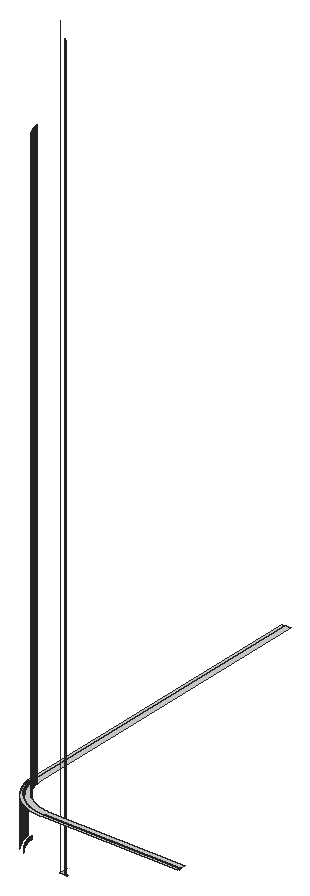
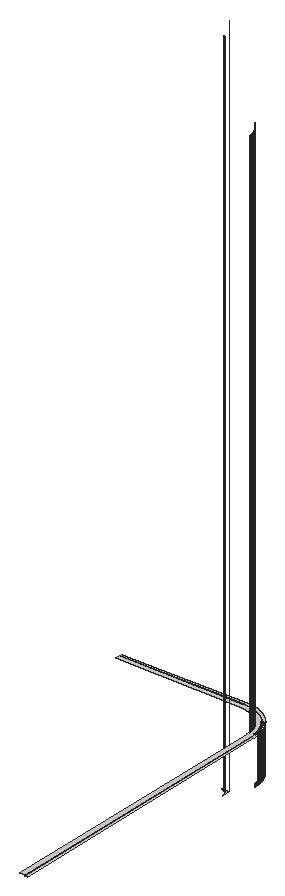
# SketchUp Ruby script. Lengths in inches.
U = 1.inch
M = Sketchup.active_model
def pt(a) = Geom::Point3d.new(a.map { |v| v * U })
def face(e, loops, mat)
  f = e.add_face(loops[0].map { |a| pt(a) })
  loops[1..].each { |l| e.add_face(l.map { |a| pt(a) }).erase! }
  f.material = f.back_material = mat if mat
  f
end
# faces: each face lists its corners as indices into pts; further lists are holes
def faces(e, pts, list, mat = nil) = list.each { |f| face(e, (f[0].is_a?(Array) ? f : [f]).map { |l| l.map { |i| pts[i] } }, mat) }
# xy, xz, yz: faces in a plane at the given z, y or x. An outline is a flat list of corners, or four numbers for a rectangle; further outlines are holes
def ring(l) = l.size == 4 ? [[l[0], l[1]], [l[2], l[1]], [l[2], l[3]], [l[0], l[3]]] : l.each_slice(2).to_a
def flat(e, list, mat, &to3) = list.each { |f| face(e, (f[0].is_a?(Array) ? f : [f]).map { |l| ring(l).map { |u, v| to3.(u, v) } }, mat) }
def xy(e, z, list, mat = nil) = flat(e, list, mat) { |x, y| [x, y, z] }
def xz(e, y, list, mat = nil) = flat(e, list, mat) { |x, z| [x, y, z] }
def yz(e, x, list, mat = nil) = flat(e, list, mat) { |y, z| [x, y, z] }
def lines(e, pts, list) = list.each { |a, b| e.add_line(pt(pts[a]), pt(pts[b])) }
# prism: a flat outline (further loops are holes) pulled along v
def prism(e, loops, v, mat = nil)
  f = face(e, loops, mat); d = Geom::Vector3d.new(v.map { |x| x * U })
  f.pushpull(f.normal.samedirection?(d) ? d.length : -d.length)
end
def box(e, o, s, mat = nil) = prism(e, [[o, [o[0] + s[0], o[1], o[2]], [o[0] + s[0], o[1] + s[1], o[2]], [o[0], o[1] + s[1], o[2]]]], [0, 0, s[2]], mat)
def at(x, y, z, deg = 0) = Geom::Transformation.translation(pt([x, y, z])) * Geom::Transformation.rotation(ORIGIN, Z_AXIS, deg.degrees)
def axes(o, x, y, z) = Geom::Transformation.new([*x, 0, *y, 0, *z, 0, *pt(o).to_a, 1])
def part(name) = M.definitions.add(name)
# library, detail: a bought-in or finely detailed component or shape, given as its bounding box
def library(name, o, s) = part(name).tap { |d| box(d.entities, o, s) }
def detail(e, o, s) = box(e.add_group.entities, o, s)
def put(e, d, t, mat = nil) = e.add_instance(d, t).tap { |i| i.material = mat if mat }
def group(e, t, mat = nil) = e.add_group.tap { |g| g.transformation = t; g.material = mat if mat }.entities
root = M.entities
M.materials.add("[Quartz Light Brown]").color = [215, 212, 212]
xy(root,126,[[213,155,213.001,157.921,213.002,157.882,213.002,157.881,213.004,157.843,213.006,157.804,213.009,157.765,213.013,157.725,213.016,157.686,213.026,157.608,213.031,157.57,213.043,157.492,213.05,157.453,213.058,157.415,213.066,157.376,213.074,157.338,213.092,157.262,213.102,157.224,213.135,157.11,213.159,157.036,213.185,156.962,213.199,156.925,213.214,156.888,213.228,156.852,213.244,156.816,213.259,156.78,213.276,156.744,213.292,156.708,213.309,156.673,213.345,156.603,213.364,156.569,213.383,156.534,213.402,156.5,213.422,156.466,213.442,156.433,213.463,156.399,213.484,156.366,213.506,156.333,213.55,156.269,213.596,156.205,213.644,156.143,213.669,156.112,213.693,156.082,213.719,156.052,213.744,156.022,213.771,155.993,213.796,155.964,213.797,155.964,213.824,155.935,213.851,155.907,213.907,155.851,213.935,155.824,213.963,155.798,213.964,155.797,213.993,155.771,214.022,155.744,214.051,155.72,214.052,155.719,214.082,155.693,214.112,155.669,214.141,155.645,214.143,155.644,214.205,155.596,214.235,155.574,214.237,155.573,214.269,155.55,214.301,155.528,214.332,155.507,214.333,155.506,214.366,155.484,214.399,155.463,214.431,155.443,214.433,155.442,214.466,155.422,214.5,155.402,214.532,155.384,214.534,155.383,214.569,155.364,214.603,155.345,214.636,155.328,214.638,155.327,214.673,155.309,214.708,155.292,214.742,155.277,214.744,155.276,214.78,155.259,214.816,155.244,214.85,155.229,214.852,155.228,214.888,155.214,214.925,155.199,214.959,155.186,214.962,155.185,215.036,155.159,215.07,155.148,215.073,155.147,215.11,155.135,215.148,155.124,215.183,155.113,215.186,155.113,215.224,155.102,215.262,155.092,215.297,155.084,215.3,155.083,215.338,155.074,215.376,155.066,215.412,155.058,215.415,155.058,215.453,155.05,215.492,155.043,215.528,155.037,215.531,155.037,215.57,155.031,215.608,155.026,215.644,155.021,215.647,155.021,215.686,155.016,215.725,155.013,215.761,155.01,215.765,155.009,215.804,155.006,215.843,155.004,215.879,155.002,215.882,155.002,215.921,155.001]],"[Quartz Light Brown]")
xy(root,149.75,[[216,143.75,263.5,143.75,263.5,144.25,216,144.25,215.82,144.251,215.64,144.255,215.46,144.261,215.28,144.269,215.101,144.279,214.921,144.292,214.742,144.308,214.563,144.325,214.384,144.345,214.205,144.368,214.027,144.392,213.849,144.419,213.671,144.449,213.494,144.48,213.318,144.514,213.141,144.55,212.965,144.589,212.79,144.63,212.615,144.673,212.441,144.719,212.268,144.766,212.095,144.816,211.923,144.868,211.751,144.923,211.58,144.98,211.41,145.039,211.241,145.1,211.072,145.163,210.905,145.229,210.738,145.297,210.572,145.367,210.407,145.439,210.243,145.513,210.08,145.589,209.919,145.668,209.758,145.749,209.598,145.831,209.439,145.916,209.281,146.003,209.125,146.092,208.97,146.183,208.816,146.276,208.663,146.371,208.511,146.468,208.361,146.567,208.212,146.668,208.064,146.771,207.918,146.876,207.773,146.983,207.63,147.091,207.487,147.202,207.347,147.314,207.208,147.428,207.07,147.544,206.934,147.662,206.799,147.782,206.666,147.903,206.535,148.026,206.405,148.151,206.277,148.277,206.151,148.405,206.026,148.535,205.903,148.666,205.782,148.799,205.662,148.934,205.544,149.07,205.428,149.208,205.314,149.347,205.202,149.487,205.091,149.63,204.983,149.773,204.876,149.918,204.771,150.064,204.668,150.212,204.567,150.361,204.468,150.511,204.371,150.663,204.276,150.816,204.183,150.97,204.092,151.125,204.003,151.281,203.916,151.439,203.831,151.598,203.749,151.758,203.668,151.919,203.589,152.08,203.513,152.243,203.439,152.407,203.367,152.572,203.297,152.738,203.229,152.905,203.163,153.072,203.1,153.241,203.039,153.41,202.98,153.58,202.923,153.751,202.868,153.923,202.816,154.095,202.766,154.268,202.719,154.441,202.673,154.615,202.63,154.79,202.589,154.965,202.55,155.141,202.514,155.318,202.48,155.494,202.449,155.671,202.419,155.849,202.392,156.027,202.368,156.205,202.345,156.384,202.325,156.563,202.308,156.742,202.292,156.921,202.279,157.101,202.269,157.28,202.261,157.46,202.255,157.64,202.251,157.82,202.25,158,202.25,266,201.75,266,201.75,158,201.751,157.813,201.755,157.627,201.761,157.441,201.77,157.254,201.781,157.068,201.794,156.882,201.81,156.696,201.828,156.51,201.849,156.325,201.872,156.14,201.897,155.955,201.925,155.771,201.956,155.587,201.989,155.403,202.024,155.22,202.061,155.037,202.101,154.855,202.144,154.673,202.188,154.492,202.236,154.312,202.285,154.132,202.337,153.953,202.391,153.774,202.447,153.597,202.506,153.419,202.567,153.243,202.631,153.068,202.696,152.893,202.764,152.72,202.835,152.547,202.907,152.375,202.982,152.204,203.059,152.034,203.138,151.865,203.22,151.697,203.303,151.531,203.389,151.365,203.477,151.2,203.567,151.037,203.659,150.875,203.753,150.714,203.85,150.554,203.948,150.396,204.049,150.239,204.152,150.083,204.256,149.929,204.363,149.776,204.472,149.624,204.582,149.474,204.695,149.325,204.809,149.178,204.926,149.032,205.044,148.888,205.164,148.745,205.286,148.604,205.41,148.465,205.536,148.327,205.663,148.191,205.793,148.056,205.924,147.924,206.056,147.793,206.191,147.663,206.327,147.536,206.465,147.41,206.604,147.286,206.745,147.164,206.888,147.044,207.032,146.926,207.178,146.809,207.325,146.695,207.474,146.582,207.624,146.472,207.776,146.363,207.929,146.256,208.083,146.152,208.239,146.049,208.396,145.948,208.554,145.85,208.714,145.753,208.875,145.659,209.037,145.567,209.2,145.477,209.365,145.389,209.531,145.303,209.697,145.22,209.865,145.138,210.034,145.059,210.204,144.982,210.375,144.907,210.547,144.835,210.72,144.764,210.893,144.696,211.068,144.631,211.243,144.567,211.419,144.506,211.597,144.447,211.774,144.391,211.953,144.337,212.132,144.285,212.312,144.236,212.492,144.188,212.673,144.144,212.855,144.101,213.037,144.061,213.22,144.024,213.403,143.989,213.587,143.956,213.771,143.925,213.955,143.897,214.14,143.872,214.325,143.849,214.51,143.828,214.696,143.81,214.882,143.794,215.068,143.781,215.254,143.77,215.441,143.761,215.627,143.755,215.813,143.751]],"[Quartz Light Brown]")
xy(root,150,[[216,143,263.5,143,263.5,143.75,216,143.75,215.813,143.751,215.627,143.755,215.441,143.761,215.254,143.77,215.068,143.781,214.882,143.794,214.696,143.81,214.51,143.828,214.325,143.849,214.14,143.872,213.955,143.897,213.771,143.925,213.587,143.956,213.403,143.989,213.22,144.024,213.037,144.061,212.855,144.101,212.673,144.144,212.492,144.188,212.312,144.236,212.132,144.285,211.953,144.337,211.774,144.391,211.597,144.447,211.419,144.506,211.243,144.567,211.068,144.631,210.893,144.696,210.72,144.764,210.547,144.835,210.375,144.907,210.204,144.982,210.034,145.059,209.865,145.138,209.697,145.22,209.531,145.303,209.365,145.389,209.2,145.477,209.037,145.567,208.875,145.659,208.714,145.753,208.554,145.85,208.396,145.948,208.239,146.049,208.083,146.152,207.929,146.256,207.776,146.363,207.624,146.472,207.474,146.582,207.325,146.695,207.178,146.809,207.032,146.926,206.888,147.044,206.745,147.164,206.604,147.286,206.465,147.41,206.327,147.536,206.191,147.663,206.056,147.793,205.924,147.924,205.793,148.056,205.663,148.191,205.536,148.327,205.41,148.465,205.286,148.604,205.164,148.745,205.044,148.888,204.926,149.032,204.809,149.178,204.695,149.325,204.582,149.474,204.472,149.624,204.363,149.776,204.256,149.929,204.152,150.083,204.049,150.239,203.948,150.396,203.85,150.554,203.753,150.714,203.659,150.875,203.567,151.037,203.477,151.2,203.389,151.365,203.303,151.531,203.22,151.697,203.138,151.865,203.059,152.034,202.982,152.204,202.907,152.375,202.835,152.547,202.764,152.72,202.696,152.893,202.631,153.068,202.567,153.243,202.506,153.419,202.447,153.597,202.391,153.774,202.337,153.953,202.285,154.132,202.236,154.312,202.188,154.492,202.144,154.673,202.101,154.855,202.061,155.037,202.024,155.22,201.989,155.403,201.956,155.587,201.925,155.771,201.897,155.955,201.872,156.14,201.849,156.325,201.828,156.51,201.81,156.696,201.794,156.882,201.781,157.068,201.77,157.254,201.761,157.441,201.755,157.627,201.751,157.813,201.75,158,201.75,266,201,266,201,158,201.001,157.804,201.005,157.607,201.012,157.411,201.021,157.215,201.032,157.019,201.046,156.823,201.063,156.627,201.082,156.432,201.104,156.237,201.128,156.042,201.155,155.848,201.185,155.653,201.217,155.46,201.251,155.266,201.288,155.074,201.328,154.881,201.37,154.69,201.414,154.498,201.462,154.308,201.511,154.118,201.563,153.928,201.618,153.74,201.675,153.552,201.734,153.365,201.796,153.178,201.86,152.993,201.927,152.808,201.996,152.624,202.068,152.442,202.142,152.26,202.218,152.079,202.297,151.899,202.378,151.72,202.461,151.542,202.547,151.366,202.635,151.19,202.725,151.016,202.818,150.843,202.913,150.671,203.01,150.5,203.109,150.331,203.21,150.163,203.314,149.996,203.42,149.83,203.528,149.666,203.638,149.504,203.75,149.343,203.865,149.183,203.981,149.025,204.1,148.869,204.22,148.714,204.343,148.56,204.467,148.408,204.594,148.258,204.722,148.11,204.853,147.963,204.985,147.818,205.119,147.675,205.255,147.533,205.393,147.393,205.533,147.255,205.675,147.119,205.818,146.985,205.963,146.853,206.11,146.722,206.258,146.594,206.408,146.467,206.56,146.343,206.714,146.22,206.869,146.1,207.025,145.981,207.183,145.865,207.343,145.75,207.504,145.638,207.666,145.528,207.83,145.42,207.996,145.314,208.163,145.21,208.331,145.109,208.5,145.01,208.671,144.913,208.843,144.818,209.016,144.725,209.19,144.635,209.366,144.547,209.542,144.461,209.72,144.378,209.899,144.297,210.079,144.218,210.26,144.142,210.442,144.068,210.624,143.996,210.808,143.927,210.993,143.86,211.178,143.796,211.365,143.734,211.552,143.675,211.74,143.618,211.928,143.563,212.118,143.511,212.308,143.462,212.498,143.414,212.69,143.37,212.881,143.328,213.074,143.288,213.266,143.251,213.46,143.217,213.653,143.185,213.848,143.155,214.042,143.128,214.237,143.104,214.432,143.082,214.627,143.063,214.823,143.046,215.019,143.032,215.215,143.021,215.411,143.012,215.607,143.005,215.804,143.001],[216,144.25,263.5,144.25,263.5,146,216,146,215.843,146.001,215.686,146.004,215.529,146.009,215.372,146.016,215.215,146.026,215.058,146.037,214.902,146.05,214.746,146.066,214.59,146.083,214.434,146.103,214.278,146.124,214.123,146.148,213.968,146.173,213.813,146.201,213.659,146.231,213.505,146.262,213.352,146.296,213.199,146.332,213.046,146.369,212.894,146.409,212.743,146.451,212.592,146.494,212.442,146.54,212.292,146.587,212.143,146.637,211.994,146.688,211.847,146.742,211.7,146.797,211.553,146.854,211.408,146.913,211.263,146.975,211.119,147.037,210.976,147.102,210.834,147.169,210.693,147.238,210.552,147.308,210.413,147.38,210.274,147.454,210.137,147.53,210,147.608,209.864,147.687,209.73,147.768,209.597,147.851,209.464,147.936,209.333,148.022,209.203,148.11,209.074,148.2,208.947,148.292,208.82,148.385,208.695,148.48,208.571,148.576,208.448,148.674,208.327,148.774,208.207,148.875,208.088,148.978,207.97,149.082,207.854,149.188,207.74,149.296,207.627,149.404,207.515,149.515,207.404,149.627,207.296,149.74,207.188,149.854,207.082,149.97,206.978,150.088,206.875,150.207,206.774,150.327,206.674,150.448,206.576,150.571,206.48,150.695,206.385,150.82,206.292,150.947,206.2,151.074,206.11,151.203,206.022,151.333,205.936,151.464,205.851,151.597,205.768,151.73,205.687,151.864,205.608,152,205.53,152.137,205.454,152.274,205.38,152.413,205.308,152.552,205.238,152.693,205.169,152.834,205.102,152.976,205.037,153.119,204.975,153.263,204.913,153.408,204.854,153.553,204.797,153.7,204.742,153.847,204.688,153.994,204.637,154.143,204.587,154.292,204.54,154.442,204.494,154.592,204.451,154.743,204.409,154.894,204.369,155.046,204.332,155.199,204.296,155.352,204.262,155.505,204.231,155.659,204.201,155.813,204.173,155.968,204.148,156.123,204.124,156.278,204.103,156.434,204.083,156.59,204.066,156.746,204.05,156.902,204.037,157.058,204.026,157.215,204.016,157.372,204.009,157.529,204.004,157.686,204.001,157.843,204,158,204,266,202.25,266,202.25,158,202.251,157.82,202.255,157.64,202.261,157.46,202.269,157.28,202.279,157.101,202.292,156.921,202.308,156.742,202.325,156.563,202.345,156.384,202.368,156.205,202.392,156.027,202.419,155.849,202.449,155.671,202.48,155.494,202.514,155.318,202.55,155.141,202.589,154.965,202.63,154.79,202.673,154.615,202.719,154.441,202.766,154.268,202.816,154.095,202.868,153.923,202.923,153.751,202.98,153.58,203.039,153.41,203.1,153.241,203.163,153.072,203.229,152.905,203.297,152.738,203.367,152.572,203.439,152.407,203.513,152.243,203.589,152.08,203.668,151.919,203.749,151.758,203.831,151.598,203.916,151.439,204.003,151.281,204.092,151.125,204.183,150.97,204.276,150.816,204.371,150.663,204.468,150.511,204.567,150.361,204.668,150.212,204.771,150.064,204.876,149.918,204.983,149.773,205.091,149.63,205.202,149.487,205.314,149.347,205.428,149.208,205.544,149.07,205.662,148.934,205.782,148.799,205.903,148.666,206.026,148.535,206.151,148.405,206.277,148.277,206.405,148.151,206.535,148.026,206.666,147.903,206.799,147.782,206.934,147.662,207.07,147.544,207.208,147.428,207.347,147.314,207.487,147.202,207.63,147.091,207.773,146.983,207.918,146.876,208.064,146.771,208.212,146.668,208.361,146.567,208.511,146.468,208.663,146.371,208.816,146.276,208.97,146.183,209.125,146.092,209.281,146.003,209.439,145.916,209.598,145.831,209.758,145.749,209.919,145.668,210.08,145.589,210.243,145.513,210.407,145.439,210.572,145.367,210.738,145.297,210.905,145.229,211.072,145.163,211.241,145.1,211.41,145.039,211.58,144.98,211.751,144.923,211.923,144.868,212.095,144.816,212.268,144.766,212.441,144.719,212.615,144.673,212.79,144.63,212.965,144.589,213.141,144.55,213.318,144.514,213.494,144.48,213.671,144.449,213.849,144.419,214.027,144.392,214.205,144.368,214.384,144.345,214.563,144.325,214.742,144.308,214.921,144.292,215.101,144.279,215.28,144.269,215.46,144.261,215.64,144.255,215.82,144.251]],"[Quartz Light Brown]")
p = [[214.78,155.259,384],[214.816,155.244,384],[214.816,155.244,126],[214.78,155.259,126],[214.569,155.364,384],[214.603,155.345,384],
  [214.603,155.345,126],[214.569,155.364,126],[214.636,155.328,384],[214.636,155.328,126],[214.638,155.327,126],[214.638,155.327,384],
  [214.673,155.309,384],[214.673,155.309,126],[214.708,155.292,384],[214.708,155.292,126],[214.742,155.277,384],[214.742,155.277,126],
  [214.744,155.276,126],[214.744,155.276,384],[214.399,155.463,384],[214.431,155.443,384],[214.431,155.443,126],[214.399,155.463,126],
  [214.433,155.442,126],[214.433,155.442,384],[214.466,155.422,384],[214.466,155.422,126],[214.5,155.402,384],[214.5,155.402,126],
  [214.532,155.384,384],[214.532,155.384,126],[214.534,155.383,126],[214.534,155.383,384],[214.269,155.55,384],[214.301,155.528,384],
  [214.301,155.528,126],[214.269,155.55,126],[214.332,155.507,384],[214.332,155.507,126],[214.333,155.506,126],[214.333,155.506,384],
  [214.366,155.484,384],[214.366,155.484,126],[214.112,155.669,384],[214.142,155.645,384],[214.141,155.645,126],[214.112,155.669,126],
  [214.143,155.644,126],[214.143,155.644,384],[214.174,155.62,384],[214.174,155.62,126],[214.205,155.596,384],[214.205,155.596,126],
  [214.235,155.574,384],[214.235,155.574,126],[214.237,155.573,126],[214.237,155.573,384],[213.993,155.771,384],[214.022,155.744,384],
  [214.022,155.744,126],[213.993,155.771,126],[214.051,155.72,384],[214.051,155.72,126],[214.052,155.719,126],[214.052,155.719,384],
  [214.082,155.693,384],[214.082,155.693,126],[213.907,155.851,384],[213.935,155.824,384],[213.935,155.824,126],[213.907,155.851,126],
  [213.963,155.798,384],[213.963,155.798,126],[213.964,155.797,126],[213.964,155.797,384],[213.797,155.964,384],[213.824,155.935,384],
  [213.824,155.935,126],[213.797,155.964,126],[213.851,155.907,384],[213.851,155.907,126],[213.878,155.88,384],[213.878,155.88,126],
  [213.879,155.879,126],[213.879,155.879,384],[213.719,156.052,384],[213.744,156.022,384],[213.744,156.022,126],[213.719,156.052,126],
  [213.771,155.993,384],[213.771,155.993,126],[213.796,155.965,384],[213.796,155.964,126],[213.62,156.174,384],[213.644,156.143,384],
  [213.644,156.143,126],[213.62,156.174,126],[213.669,156.112,384],[213.669,156.112,126],[213.693,156.082,384],[213.693,156.082,126],
  [213.55,156.269,384],[213.573,156.237,384],[213.573,156.237,126],[213.55,156.269,126],[213.596,156.205,384],[213.596,156.205,126],
  [213.528,156.301,384],[213.528,156.301,126],[205.12,149.19,133],[205.12,149.19,132],[205.236,149.048,132],[205.236,149.048,133],
  [205.006,149.333,133],[205.006,149.333,132],[204.893,149.477,133],[204.893,149.477,132],[204.782,149.623,133],[204.782,149.623,132],
  [204.674,149.771,133],[204.674,149.771,132],[204.567,149.92,133],[204.567,149.92,132],[204.462,150.07,133],[204.462,150.07,132],
  [204.359,150.222,133],[204.359,150.222,132],[204.259,150.375,133],[204.259,150.375,132],[204.16,150.529,133],[204.16,150.529,132],
  [204.063,150.685,133],[204.063,150.685,132],[203.968,150.842,133],[203.968,150.842,132],[203.876,151,133],[203.876,151,132],
  [203.785,151.159,133],[203.785,151.159,132],[203.697,151.32,133],[203.697,151.32,132],[203.61,151.481,133],[203.61,151.481,132],
  [203.526,151.644,133],[203.526,151.644,132],[203.444,151.808,133],[203.444,151.808,132],[203.364,151.973,133],[203.364,151.973,132],
  [203.286,152.139,133],[203.286,152.139,132],[203.21,152.306,133],[203.21,152.306,132],[203.137,152.474,133],[203.137,152.474,132],
  [203.066,152.642,133],[203.066,152.642,132],[202.997,152.812,133],[202.997,152.812,132],[202.93,152.983,133],[202.93,152.983,132],
  [202.865,153.154,133],[202.865,153.154,132],[202.803,153.327,133],[202.803,153.327,132],[202.743,153.5,133],[202.743,153.5,132],
  [202.685,153.674,133],[202.685,153.674,132],[202.63,153.848,133],[202.63,153.848,132],[202.577,154.024,133],[202.577,154.024,132],
  [202.526,154.2,133],[202.526,154.2,132],[202.477,154.377,133],[202.477,154.377,132],[202.431,154.554,133],[202.431,154.554,132],
  [202.387,154.732,133],[202.387,154.732,132],[202.345,154.91,133],[202.345,154.91,132],[202.306,155.089,133],[202.306,155.089,132],
  [202.269,155.269,133],[202.269,155.269,132],[202.234,155.449,133],[202.234,155.449,132],[202.202,155.629,133],[202.202,155.629,132],
  [202.172,155.81,133],[202.172,155.81,132],[202.145,155.991,133],[202.145,155.991,132],[202.12,156.173,133],[202.12,156.173,132],
  [202.097,156.354,133],[202.097,156.354,132],[203.981,149.025,133],[203.981,149.025,150],[203.865,149.183,150],[203.865,149.183,133],
  [203.75,149.343,150],[203.75,149.343,133],[203.638,149.504,150],[203.638,149.504,133],[203.528,149.666,150],[203.528,149.666,133],
  [203.42,149.83,150],[203.42,149.83,133],[203.314,149.996,150],[203.314,149.996,133],[203.21,150.163,150],[203.21,150.163,133],
  [203.109,150.331,150],[203.109,150.331,133],[203.01,150.5,150],[203.01,150.5,133],[202.913,150.671,150],[202.913,150.671,133],
  [202.818,150.843,150],[202.818,150.843,133],[202.725,151.016,150],[202.725,151.016,133],[202.635,151.19,150],[202.635,151.19,133],
  [202.547,151.366,150],[202.547,151.366,133],[202.461,151.542,150],[202.461,151.542,133],[202.378,151.72,150],[202.378,151.72,133],
  [202.297,151.899,150],[202.297,151.899,133],[202.218,152.079,150],[202.218,152.079,133],[202.142,152.26,150],[202.142,152.26,133],
  [202.068,152.442,150],[202.068,152.442,133],[201.996,152.624,150],[201.996,152.624,133],[201.927,152.808,150],[201.927,152.808,133],
  [201.86,152.993,150],[201.86,152.993,133],[201.796,153.178,150],[201.796,153.178,133],[201.734,153.365,150],[201.734,153.365,133],
  [201.675,153.552,150],[201.675,153.552,133],[201.618,153.74,150],[201.618,153.74,133],[201.563,153.928,150],[201.563,153.928,133],
  [201.511,154.118,150],[201.511,154.118,133],[201.462,154.308,150],[201.462,154.308,133],[201.414,154.498,150],[201.414,154.498,133],
  [201.37,154.69,150],[201.37,154.69,133],[201.328,154.881,150],[201.328,154.881,133],[201.288,155.074,150],[201.288,155.074,133],
  [201.251,155.266,150],[201.251,155.266,133],[201.217,155.46,150],[201.217,155.46,133],[201.185,155.653,150],[201.185,155.653,133],
  [201.155,155.848,150],[201.155,155.848,133],[201.128,156.042,150],[201.128,156.042,133],[201.104,156.237,150],[201.104,156.237,133],
  [205.662,148.934,150],[205.544,149.07,150],[205.544,149.07,149.75],[205.662,148.934,149.75],[204.809,149.178,150],[204.926,149.032,150],
  [204.926,149.032,149.75],[204.809,149.178,149.75],[205.428,149.208,150],[205.428,149.208,149.75],[204.695,149.325,150],[204.695,149.325,149.75],
  [205.314,149.347,150],[205.314,149.347,149.75],[204.582,149.474,150],[204.582,149.474,149.75],[205.202,149.487,150],[205.202,149.487,149.75],
  [204.472,149.624,150],[204.472,149.624,149.75],[205.091,149.63,150],[205.091,149.63,149.75],[204.363,149.776,150],[204.363,149.776,149.75],
  [204.983,149.773,150],[204.983,149.773,149.75],[204.256,149.929,150],[204.256,149.929,149.75],[204.876,149.918,150],[204.876,149.918,149.75],
  [204.152,150.083,150],[204.152,150.083,149.75],[204.771,150.064,150],[204.771,150.064,149.75],[204.049,150.239,150],[204.049,150.239,149.75],
  [204.668,150.212,150],[204.668,150.212,149.75],[203.948,150.396,150],[203.948,150.396,149.75],[204.567,150.361,150],[204.567,150.361,149.75],
  [203.85,150.554,150],[203.85,150.554,149.75],[204.468,150.511,150],[204.468,150.511,149.75],[204.371,150.663,150],[204.371,150.663,149.75],
  [203.753,150.714,150],[203.753,150.714,149.75],[203.659,150.875,150],[203.659,150.875,149.75],[204.276,150.816,150],[204.276,150.816,149.75],
  [204.183,150.97,150],[204.183,150.97,149.75],[203.567,151.037,150],[203.567,151.037,149.75],[203.477,151.2,150],[203.477,151.2,149.75],
  [204.092,151.125,150],[204.092,151.125,149.75],[204.003,151.281,150],[204.003,151.281,149.75],[203.389,151.365,150],[203.389,151.365,149.75],
  [203.916,151.439,150],[203.916,151.439,149.75],[203.303,151.531,150],[203.303,151.531,149.75],[203.831,151.598,150],[203.831,151.598,149.75],
  [203.22,151.697,150],[203.22,151.697,149.75],[203.749,151.758,150],[203.749,151.758,149.75],[203.138,151.865,150],[203.138,151.865,149.75],
  [203.668,151.919,150],[203.668,151.919,149.75],[203.059,152.034,150],[203.059,152.034,149.75],[203.589,152.08,150],[203.589,152.08,149.75],
  [202.982,152.204,150],[202.982,152.204,149.75],[203.513,152.243,150],[203.513,152.243,149.75],[202.907,152.375,150],[202.907,152.375,149.75],
  [203.439,152.407,150],[203.439,152.407,149.75],[202.835,152.547,150],[202.835,152.547,149.75],[203.367,152.572,150],[203.367,152.572,149.75],
  [202.764,152.72,150],[202.764,152.72,149.75],[203.297,152.738,150],[203.297,152.738,149.75],[202.696,152.893,150],[202.696,152.893,149.75],
  [203.229,152.905,150],[203.229,152.905,149.75],[202.631,153.068,150],[202.631,153.068,149.75],[203.163,153.072,150],[203.163,153.072,149.75],
  [202.567,153.243,150],[202.567,153.243,149.75],[203.1,153.241,150],[203.1,153.241,149.75],[202.506,153.419,150],[202.506,153.419,149.75],
  [203.039,153.41,150],[203.039,153.41,149.75],[202.447,153.597,150],[202.447,153.597,149.75],[202.98,153.58,150],[202.98,153.58,149.75],
  [202.391,153.774,150],[202.391,153.774,149.75],[202.923,153.751,150],[202.923,153.751,149.75],[202.337,153.953,150],[202.337,153.953,149.75],
  [202.868,153.923,150],[202.868,153.923,149.75],[202.816,154.095,150],[202.816,154.095,149.75],[202.285,154.132,150],[202.285,154.132,149.75],
  [202.236,154.312,150],[202.236,154.312,149.75],[202.766,154.268,150],[202.766,154.268,149.75],[202.188,154.492,150],[202.188,154.492,149.75],
  [202.719,154.441,150],[202.719,154.441,149.75],[202.673,154.615,150],[202.673,154.615,149.75],[202.144,154.673,150],[202.144,154.673,149.75],
  [202.63,154.79,150],[202.63,154.79,149.75],[202.101,154.855,150],[202.101,154.855,149.75],[202.589,154.965,150],[202.589,154.965,149.75],
  [202.061,155.037,150],[202.061,155.037,149.75],[202.024,155.22,150],[202.024,155.22,149.75],[202.55,155.141,150],[202.55,155.141,149.75],
  [202.514,155.318,150],[202.514,155.318,149.75],[201.989,155.403,150],[201.989,155.403,149.75],[202.48,155.494,150],[202.48,155.494,149.75],
  [201.956,155.587,150],[201.956,155.587,149.75],[202.449,155.671,150],[202.449,155.671,149.75],[201.925,155.771,150],[201.925,155.771,149.75],
  [202.419,155.849,150],[202.419,155.849,149.75],[201.897,155.955,150],[201.897,155.955,149.75],[202.392,156.027,150],[202.392,156.027,149.75],
  [201.872,156.14,150],[201.872,156.14,149.75],[202.368,156.205,150],[202.368,156.205,149.75],[201.849,156.325,150],[201.849,156.325,149.75],
  [202.345,156.384,150],[202.345,156.384,149.75],[208.088,148.978,150],[208.088,148.978,354],[207.97,149.082,354],[207.97,149.082,150],
  [207.854,149.188,354],[207.854,149.188,150],[207.74,149.296,354],[207.74,149.296,150],[207.627,149.404,354],[207.627,149.404,150],
  [207.515,149.515,354],[207.515,149.515,150],[207.404,149.627,354],[207.404,149.627,150],[207.296,149.74,354],[207.296,149.74,150],
  [207.188,149.854,354],[207.188,149.854,150],[207.082,149.97,354],[207.082,149.97,150],[206.978,150.088,354],[206.978,150.088,150],
  [206.875,150.207,354],[206.875,150.207,150],[206.774,150.327,354],[206.774,150.327,150],[206.674,150.448,354],[206.674,150.448,150],
  [206.576,150.571,354],[206.576,150.571,150],[206.48,150.695,354],[206.48,150.695,150],[206.385,150.82,354],[206.385,150.82,150],
  [206.292,150.947,354],[206.292,150.947,150],[206.2,151.074,354],[206.2,151.074,150],[206.11,151.203,354],[206.11,151.203,150],
  [206.022,151.333,354],[206.022,151.333,150],[205.936,151.464,354],[205.936,151.464,150],[205.851,151.597,354],[205.851,151.597,150],
  [205.768,151.73,354],[205.768,151.73,150],[205.687,151.864,354],[205.687,151.864,150],[205.608,152,354],[205.608,152,150],
  [205.53,152.137,354],[205.53,152.137,150],[205.454,152.274,354],[205.454,152.274,150],[205.38,152.413,354],[205.38,152.413,150],
  [205.308,152.552,354],[205.308,152.552,150],[205.238,152.693,354],[205.238,152.693,150],[205.169,152.834,354],[205.169,152.834,150],
  [205.102,152.976,354],[205.102,152.976,150],[205.037,153.119,354],[205.037,153.119,150],[204.975,153.263,354],[204.975,153.263,150],
  [204.913,153.408,354],[204.913,153.408,150],[204.854,153.553,354],[204.854,153.553,150],[204.797,153.7,354],[204.797,153.7,150],
  [204.742,153.847,354],[204.742,153.847,150],[204.688,153.994,354],[204.688,153.994,150],[204.637,154.143,354],[204.637,154.143,150],
  [204.587,154.292,354],[204.587,154.292,150],[204.54,154.442,354],[204.54,154.442,150],[204.494,154.592,354],[204.494,154.592,150],
  [204.451,154.743,354],[204.451,154.743,150],[204.409,154.894,354],[204.409,154.894,150],[204.369,155.046,354],[204.369,155.046,150],
  [204.332,155.199,354],[204.332,155.199,150],[204.296,155.352,354],[204.296,155.352,150],[204.262,155.505,354],[204.262,155.505,150],
  [204.231,155.659,354],[204.231,155.659,150],[204.201,155.813,354],[204.201,155.813,150],[204.173,155.968,354],[204.173,155.968,150],
  [204.148,156.123,354],[204.148,156.123,150],[204.124,156.278,354],[204.124,156.278,150],[213,155,126],[213,155,390]]
faces(root,p,[[0,1,2,3],[4,5,6,7],[5,8,9,6],[10,9,8,11],[11,12,13,10],[12,14,15,13],[14,16,17,15],[18,17,16,19],
  [19,0,3,18],[20,21,22,23],[24,22,21,25],[25,26,27,24],[26,28,29,27],[28,30,31,29],[32,31,30,33],[33,4,7,32],
  [34,35,36,37],[35,38,39,36],[40,39,38,41],[41,42,43,40],[42,20,23,43],[44,45,46,47],[48,46,45,49],[49,50,51,48],
  [50,52,53,51],[52,54,55,53],[56,55,54,57],[57,34,37,56],[58,59,60,61],[59,62,63,60],[64,63,62,65],[65,66,67,64],
  [66,44,47,67],[68,69,70,71],[69,72,73,70],[74,73,72,75],[75,58,61,74],[76,77,78,79],[77,80,81,78],[80,82,83,81],
  [84,83,82,85],[85,68,71,84],[86,87,88,89],[87,90,91,88],[90,92,93,91],[79,93,92,76],[94,95,96,97],[95,98,99,96],
  [98,100,101,99],[100,86,89,101],[102,103,104,105],[103,106,107,104],[106,94,97,107],[108,102,105,109],[110,111,112,113],[114,115,111,110],
  [116,117,115,114],[118,119,117,116],[120,121,119,118],[122,123,121,120],[124,125,123,122],[126,127,125,124],[128,129,127,126],[130,131,129,128],
  [132,133,131,130],[134,135,133,132],[136,137,135,134],[138,139,137,136],[140,141,139,138],[142,143,141,140],[144,145,143,142],[146,147,145,144],
  [148,149,147,146],[150,151,149,148],[152,153,151,150],[154,155,153,152],[156,157,155,154],[158,159,157,156],[160,161,159,158],[162,163,161,160],
  [164,165,163,162],[166,167,165,164],[168,169,167,166],[170,171,169,168],[172,173,171,170],[174,175,173,172],[176,177,175,174],[178,179,177,176],
  [180,181,179,178],[182,183,181,180],[184,185,183,182],[186,187,185,184],[188,189,187,186],[190,191,189,188],[192,193,191,190],[194,195,193,192],
  [196,197,195,194],[198,199,197,196],[200,201,202,203],[203,202,204,205],[205,204,206,207],[207,206,208,209],[209,208,210,211],[211,210,212,213],
  [213,212,214,215],[215,214,216,217],[217,216,218,219],[219,218,220,221],[221,220,222,223],[223,222,224,225],[225,224,226,227],[227,226,228,229],
  [229,228,230,231],[231,230,232,233],[233,232,234,235],[235,234,236,237],[237,236,238,239],[239,238,240,241],[241,240,242,243],[243,242,244,245],
  [245,244,246,247],[247,246,248,249],[249,248,250,251],[251,250,252,253],[253,252,254,255],[255,254,256,257],[257,256,258,259],[259,258,260,261],
  [261,260,262,263],[263,262,264,265],[265,264,266,267],[267,266,268,269],[269,268,270,271],[271,270,272,273],[273,272,274,275],[275,274,276,277],
  [277,276,278,279],[279,278,280,281],[282,283,284,285],[286,287,288,289],[283,290,291,284],[292,286,289,293],[290,294,295,291],[296,292,293,297],
  [294,298,299,295],[300,296,297,301],[298,302,303,299],[304,300,301,305],[302,306,307,303],[308,304,305,309],[306,310,311,307],[312,308,309,313],
  [310,314,315,311],[316,312,313,317],[314,318,319,315],[320,316,317,321],[318,322,323,319],[324,320,321,325],[322,326,327,323],[326,328,329,327],
  [330,324,325,331],[332,330,331,333],[328,334,335,329],[334,336,337,335],[338,332,333,339],[340,338,339,341],[336,342,343,337],[342,344,345,343],
  [346,340,341,347],[344,348,349,345],[350,346,347,351],[348,352,353,349],[354,350,351,355],[352,356,357,353],[358,354,355,359],[356,360,361,357],
  [362,358,359,363],[360,364,365,361],[366,362,363,367],[364,368,369,365],[370,366,367,371],[368,372,373,369],[374,370,371,375],[372,376,377,373],
  [378,374,375,379],[376,380,381,377],[382,378,379,383],[380,384,385,381],[386,382,383,387],[384,388,389,385],[390,386,387,391],[388,392,393,389],
  [394,390,391,395],[392,396,397,393],[398,394,395,399],[396,400,401,397],[402,398,399,403],[400,404,405,401],[406,402,403,407],[404,408,409,405],
  [408,410,411,409],[412,406,407,413],[414,412,413,415],[410,416,417,411],[418,414,415,419],[416,420,421,417],[420,422,423,421],[424,418,419,425],
  [422,426,427,423],[428,424,425,429],[426,430,431,427],[432,428,429,433],[434,432,433,435],[430,436,437,431],[436,438,439,437],[440,434,435,441],
  [438,442,443,439],[444,440,441,445],[442,446,447,443],[448,444,445,449],[446,450,451,447],[452,448,449,453],[450,454,455,451],[456,452,453,457],
  [454,458,459,455],[460,456,457,461],[458,462,463,459],[464,465,466,467],[467,466,468,469],[469,468,470,471],[471,470,472,473],[473,472,474,475],
  [475,474,476,477],[477,476,478,479],[479,478,480,481],[481,480,482,483],[483,482,484,485],[485,484,486,487],[487,486,488,489],[489,488,490,491],
  [491,490,492,493],[493,492,494,495],[495,494,496,497],[497,496,498,499],[499,498,500,501],[501,500,502,503],[503,502,504,505],[505,504,506,507],
  [507,506,508,509],[509,508,510,511],[511,510,512,513],[513,512,514,515],[515,514,516,517],[517,516,518,519],[519,518,520,521],[521,520,522,523],
  [523,522,524,525],[525,524,526,527],[527,526,528,529],[529,528,530,531],[531,530,532,533],[533,532,534,535],[535,534,536,537],[537,536,538,539],
  [539,538,540,541],[541,540,542,543],[543,542,544,545],[545,544,546,547],[547,546,548,549],[549,548,550,551],[551,550,552,553],[553,552,554,555],
  [555,554,556,557],[557,556,558,559],[559,558,560,561],[561,560,562,563],[563,562,564,565],[565,564,566,567],[567,566,568,569],[569,568,570,571],
  [571,570,572,573]],"[Quartz Light Brown]")
lines(root,p,[[574,575]])
